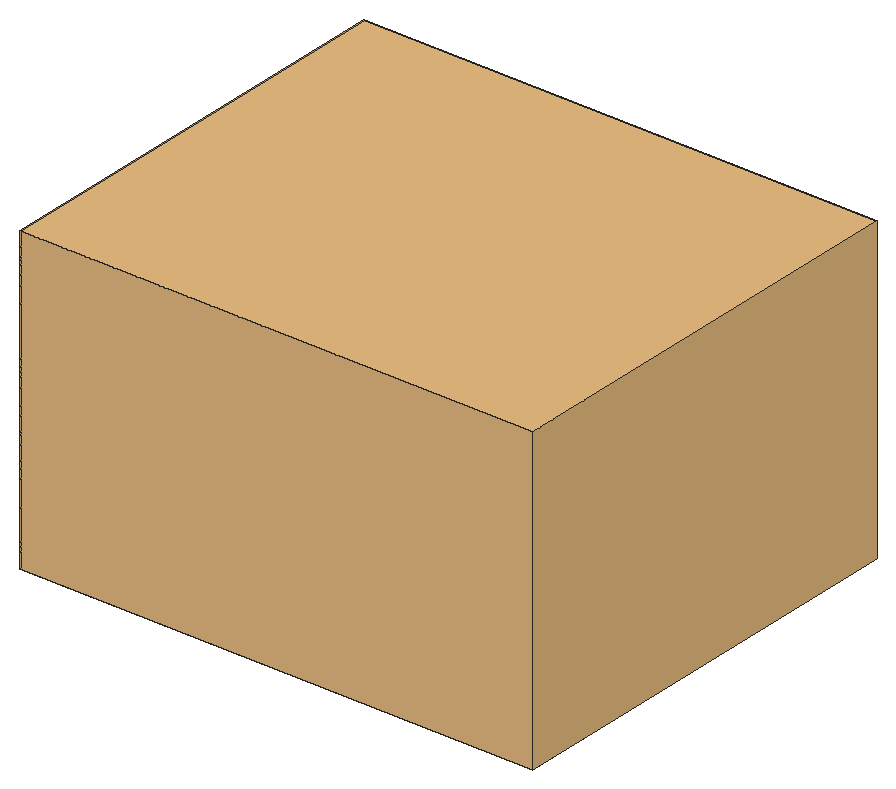
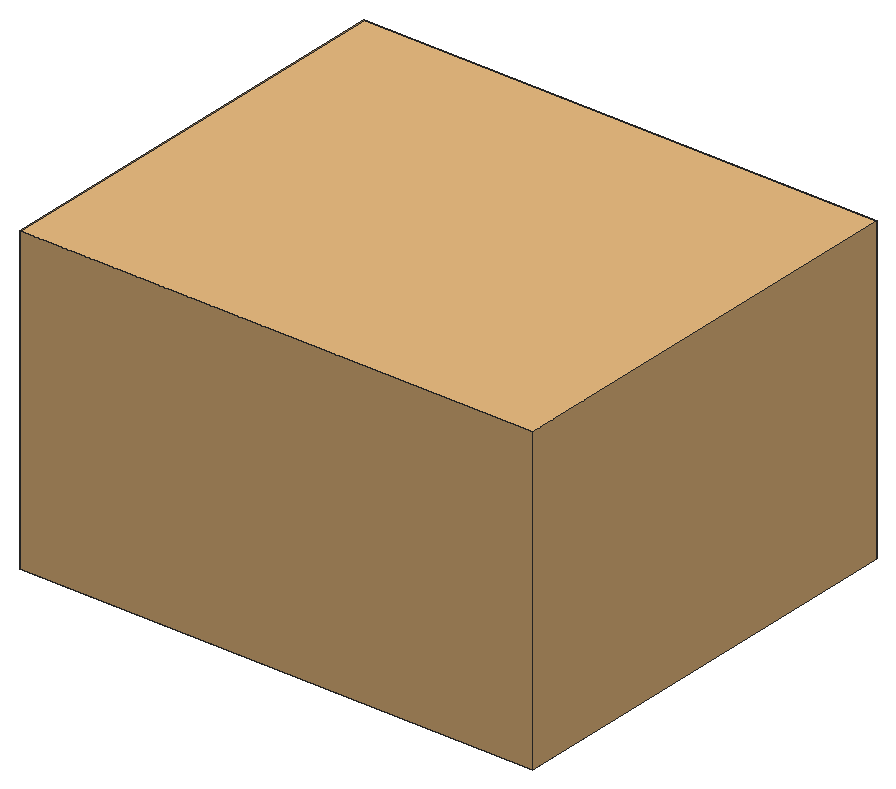
# SketchUp Ruby script. Lengths in inches.
U = 1.inch
M = Sketchup.active_model
def pt(a) = Geom::Point3d.new(a.map { |v| v * U })
def face(e, loops, mat)
  f = e.add_face(loops[0].map { |a| pt(a) })
  loops[1..].each { |l| e.add_face(l.map { |a| pt(a) }).erase! }
  f.material = f.back_material = mat if mat
  f
end
# faces: each face lists its corners as indices into pts; further lists are holes
def faces(e, pts, list, mat = nil) = list.each { |f| face(e, (f[0].is_a?(Array) ? f : [f]).map { |l| l.map { |i| pts[i] } }, mat) }
# xy, xz, yz: faces in a plane at the given z, y or x. An outline is a flat list of corners, or four numbers for a rectangle; further outlines are holes
def ring(l) = l.size == 4 ? [[l[0], l[1]], [l[2], l[1]], [l[2], l[3]], [l[0], l[3]]] : l.each_slice(2).to_a
def flat(e, list, mat, &to3) = list.each { |f| face(e, (f[0].is_a?(Array) ? f : [f]).map { |l| ring(l).map { |u, v| to3.(u, v) } }, mat) }
def xy(e, z, list, mat = nil) = flat(e, list, mat) { |x, y| [x, y, z] }
def xz(e, y, list, mat = nil) = flat(e, list, mat) { |x, z| [x, y, z] }
def yz(e, x, list, mat = nil) = flat(e, list, mat) { |y, z| [x, y, z] }
def lines(e, pts, list) = list.each { |a, b| e.add_line(pt(pts[a]), pt(pts[b])) }
# prism: a flat outline (further loops are holes) pulled along v
def prism(e, loops, v, mat = nil)
  f = face(e, loops, mat); d = Geom::Vector3d.new(v.map { |x| x * U })
  f.pushpull(f.normal.samedirection?(d) ? d.length : -d.length)
end
def box(e, o, s, mat = nil) = prism(e, [[o, [o[0] + s[0], o[1], o[2]], [o[0] + s[0], o[1] + s[1], o[2]], [o[0], o[1] + s[1], o[2]]]], [0, 0, s[2]], mat)
def at(x, y, z, deg = 0) = Geom::Transformation.translation(pt([x, y, z])) * Geom::Transformation.rotation(ORIGIN, Z_AXIS, deg.degrees)
def axes(o, x, y, z) = Geom::Transformation.new([*x, 0, *y, 0, *z, 0, *pt(o).to_a, 1])
def part(name) = M.definitions.add(name)
# library, detail: a bought-in or finely detailed component or shape, given as its bounding box
def library(name, o, s) = part(name).tap { |d| box(d.entities, o, s) }
def detail(e, o, s) = box(e.add_group.entities, o, s)
def put(e, d, t, mat = nil) = e.add_instance(d, t).tap { |i| i.material = mat if mat }
def group(e, t, mat = nil) = e.add_group.tap { |g| g.transformation = t; g.material = mat if mat }.entities
root = M.entities
M.materials.add("1432 AP 8245 TAR ROAD").color = [57, 57, 60]
c1 = library("Group\#17",[-9,-12.5,-6],[243.5,204.5,144])
xz(root,255.5,[[189.84,108,189.92,111],[189.92,108,190,111],[190,108,190.08,111],[190.08,108,190.16,111],[259.34,108,259.42,111],
  [259.42,108,259.5,111],[259.5,108,259.58,111],[259.58,108,259.66,111]])
xz(root,314,[[259.34,108,259.42,111],[259.42,108,259.5,111],[259.5,108,259.58,111],[259.58,108,259.66,111]])
xz(root,320,[[259.34,108,259.42,111],[259.42,108,259.5,111],[259.5,108,259.58,111],[259.58,108,259.66,111]])
yz(root,193,[[252.34,108,252.42,111],[252.42,108,252.5,111],[252.5,108,252.58,111],[252.58,108,252.66,111]])
yz(root,213,[[275,107.5,335,108.5]])
yz(root,215,[[273,108,333,108.5]])
yz(root,256.5,[[252.34,108,252.42,111],[252.42,108,252.5,111],[252.5,108,252.58,111],[252.58,108,252.66,111],[316.84,108,316.92,111],
  [316.92,108,317,111],[317,108,317.08,111],[317.08,108,317.16,111]])
p = [[191.76,250.07,108],[191.7,250.03,108],[191.7,250.03,111],[191.76,250.07,111],[191.83,250.12,108],[191.83,250.12,111],
  [191.89,250.17,108],[191.89,250.17,111],[257.67,250.12,108],[257.61,250.17,108],[257.61,250.17,111],[257.67,250.12,111],
  [257.74,250.07,108],[257.74,250.07,111],[191.95,250.22,108],[191.95,250.22,111],[192.01,250.27,108],[192.01,250.27,111],
  [257.55,250.22,108],[257.49,250.27,108],[257.49,250.27,111],[257.55,250.22,111],[192.07,250.32,108],[192.07,250.32,111],
  [192.12,250.38,108],[192.12,250.38,111],[257.43,250.32,108],[257.43,250.32,111],[257.38,250.38,108],[257.38,250.38,111],
  [192.18,250.43,108],[192.18,250.43,111],[192.23,250.49,108],[192.23,250.49,111],[257.32,250.43,108],[257.32,250.43,111],
  [257.27,250.49,108],[257.27,250.49,111],[192.28,250.55,108],[192.28,250.55,111],[257.22,250.55,108],[257.22,250.55,111],
  [192.33,250.61,108],[192.33,250.61,111],[192.38,250.67,108],[192.38,250.67,111],[257.17,250.61,108],[257.12,250.67,108],
  [257.12,250.67,111],[257.17,250.61,111],[192.43,250.74,108],[192.43,250.74,111],[192.47,250.8,108],[192.47,250.8,111],
  [257.07,250.74,108],[257.03,250.8,108],[257.03,250.8,111],[257.07,250.74,111],[192.52,250.87,108],[192.52,250.87,111],
  [256.98,250.87,108],[256.98,250.87,111],[192.56,250.93,108],[192.56,250.93,111],[192.6,251,108],[192.6,251,111],
  [256.94,250.93,108],[256.94,250.93,111],[256.9,251,108],[256.9,251,111],[192.64,251.07,108],[192.64,251.07,111],
  [256.86,251.07,108],[256.86,251.07,111],[192.67,251.14,108],[192.67,251.14,111],[192.71,251.21,108],[192.71,251.21,111],
  [256.83,251.14,108],[256.83,251.14,111],[256.79,251.21,108],[256.79,251.21,111],[192.74,251.28,108],[192.74,251.28,111],
  [256.76,251.28,108],[256.76,251.28,111],[192.77,251.35,108],[192.77,251.35,111],[256.73,251.35,108],[256.73,251.35,111],
  [192.8,251.42,108],[192.8,251.42,111],[192.83,251.5,108],[192.83,251.5,111],[256.7,251.42,108],[256.7,251.42,111],
  [256.67,251.5,108],[256.67,251.5,111],[192.85,251.57,108],[192.85,251.57,111],[256.65,251.57,108],[256.65,251.57,111],
  [192.875,251.65,108],[192.875,251.65,111],[192.9,251.72,108],[192.9,251.72,111],[256.625,251.65,108],[256.625,251.65,111],
  [256.6,251.72,108],[256.6,251.72,111],[192.92,251.8,108],[192.92,251.8,111],[256.58,251.8,108],[256.58,251.8,111],
  [192.93,251.875,108],[192.93,251.875,111],[256.57,251.875,108],[256.57,251.875,111],[192.95,251.95,108],[192.95,251.95,111],
  [256.55,251.95,108],[256.55,251.95,111],[192.96,252.03,108],[192.96,252.03,111],[192.97,252.11,108],[192.97,252.11,111],
  [256.54,252.03,108],[256.54,252.03,111],[256.53,252.11,108],[256.53,252.11,111],[192.98,252.1875,108],[192.98,252.1875,111],
  [256.52,252.1875,108],[256.52,252.1875,111],[192.99,252.26,108],[192.99,252.26,111],[256.51,252.26,108],[256.51,252.26,111],
  [193,252.34,108],[193,252.34,111],[256.5,252.34,108],[256.5,252.34,111],[192.99,252.74,108],[193,252.66,108],
  [193,252.66,111],[192.99,252.74,111],[192.98,252.8125,108],[192.98,252.8125,111],[256.5,252.66,108],[256.51,252.74,108],
  [256.51,252.74,111],[256.5,252.66,111],[256.52,252.8125,108],[256.52,252.8125,111],[192.97,252.89,108],[192.97,252.89,111],
  [256.53,252.89,108],[256.53,252.89,111],[192.96,252.97,108],[192.96,252.97,111],[256.54,252.97,108],[256.54,252.97,111],
  [192.95,253.05,108],[192.95,253.05,111],[192.93,253.125,108],[192.93,253.125,111],[256.55,253.05,108],[256.55,253.05,111],
  [256.57,253.125,108],[256.57,253.125,111],[192.92,253.2,108],[192.92,253.2,111],[256.58,253.2,108],[256.58,253.2,111],
  [192.9,253.28,108],[192.9,253.28,111],[256.6,253.28,108],[256.6,253.28,111],[192.875,253.35,108],[192.875,253.35,111],
  [256.625,253.35,108],[256.625,253.35,111],[192.83,253.5,108],[192.85,253.43,108],[192.85,253.43,111],[192.83,253.5,111],
  [256.65,253.43,108],[256.65,253.43,111],[256.67,253.5,108],[256.67,253.5,111],[192.8,253.58,108],[192.8,253.58,111],
  [256.7,253.58,108],[256.7,253.58,111],[192.74,253.72,108],[192.77,253.65,108],[192.77,253.65,111],[192.74,253.72,111],
  [256.73,253.65,108],[256.73,253.65,111],[256.76,253.72,108],[256.76,253.72,111],[192.71,253.79,108],[192.71,253.79,111],
  [256.79,253.79,108],[256.79,253.79,111],[192.67,253.86,108],[192.67,253.86,111],[256.83,253.86,108],[256.83,253.86,111],
  [192.64,253.93,108],[192.64,253.93,111],[192.6,254,108],[192.6,254,111],[256.86,253.93,108],[256.86,253.93,111],
  [256.9,254,108],[256.9,254,111],[192.56,254.07,108],[192.56,254.07,111],[256.94,254.07,108],[256.94,254.07,111],
  [192.52,254.13,108],[192.52,254.13,111],[192.47,254.2,108],[192.47,254.2,111],[256.98,254.13,108],[256.98,254.13,111],
  [257.03,254.2,108],[257.03,254.2,111],[192.43,254.26,108],[192.43,254.26,111],[257.07,254.26,108],[257.07,254.26,111],
  [192.33,254.39,108],[192.38,254.33,108],[192.38,254.33,111],[192.33,254.39,111],[257.12,254.33,108],[257.12,254.33,111],
  [257.17,254.39,108],[257.17,254.39,111],[192.23,254.51,108],[192.28,254.45,108],[192.28,254.45,111],[192.23,254.51,111],
  [257.22,254.45,108],[257.22,254.45,111],[257.27,254.51,108],[257.27,254.51,111],[192.18,254.57,108],[192.18,254.57,111],
  [257.32,254.57,108],[257.32,254.57,111],[192.12,254.62,108],[192.12,254.62,111],[192.07,254.68,108],[192.07,254.68,111],
  [257.38,254.62,108],[257.38,254.62,111],[257.43,254.68,108],[257.43,254.68,111],[191.95,254.78,108],[192.01,254.73,108],
  [192.01,254.73,111],[191.95,254.78,111],[257.49,254.73,108],[257.49,254.73,111],[257.55,254.78,108],[257.55,254.78,111],
  [191.83,254.88,108],[191.89,254.83,108],[191.89,254.83,111],[191.83,254.88,111],[257.61,254.83,108],[257.61,254.83,111],
  [257.67,254.88,108],[257.67,254.88,111],[191.7,254.97,108],[191.76,254.93,108],[191.76,254.93,111],[191.7,254.97,111],
  [257.74,254.93,108],[257.74,254.93,111],[257.8,254.97,108],[257.8,254.97,111],[191.63,255.02,108],[191.63,255.02,111],
  [191.57,255.06,108],[191.57,255.06,111],[257.87,255.02,108],[257.87,255.02,111],[257.93,255.06,108],[257.93,255.06,111],
  [191.43,255.14,108],[191.5,255.1,108],[191.5,255.1,111],[191.43,255.14,111],[191.36,255.17,108],[191.36,255.17,111],
  [258,255.1,108],[258,255.1,111],[258.07,255.14,108],[258.07,255.14,111],[258.14,255.17,108],[258.14,255.17,111],
  [191.15,255.27,108],[191.22,255.24,108],[191.22,255.24,111],[191.15,255.27,111],[191.29,255.21,108],[191.29,255.21,111],
  [258.21,255.21,108],[258.21,255.21,111],[258.28,255.24,108],[258.28,255.24,111],[258.35,255.27,108],[258.35,255.27,111],
  [190.93,255.35,108],[191,255.33,108],[191,255.33,111],[190.93,255.35,111],[191.08,255.3,108],[191.08,255.3,111],
  [258.42,255.3,108],[258.42,255.3,111],[258.5,255.33,108],[258.5,255.33,111],[258.57,255.35,108],[258.57,255.35,111],
  [189.15,255.375,108],[189.22,255.4,108],[189.22,255.4,111],[189.15,255.375,111],[189.3,255.42,108],[189.3,255.42,111],
  [189.375,255.43,108],[189.375,255.43,111],[189.45,255.45,108],[189.45,255.45,111],[189.53,255.46,108],[189.53,255.46,111],
  [190.55,255.45,108],[190.625,255.43,108],[190.625,255.43,111],[190.55,255.45,111],[190.47,255.46,108],[190.47,255.46,111],
  [190.7,255.42,108],[190.7,255.42,111],[190.78,255.4,108],[190.78,255.4,111],[190.85,255.375,108],[190.85,255.375,111],
  [258.65,255.375,108],[258.65,255.375,111],[258.72,255.4,108],[258.72,255.4,111],[258.8,255.42,108],[258.8,255.42,111],
  [258.875,255.43,108],[258.875,255.43,111],[258.95,255.45,108],[258.95,255.45,111],[259.03,255.46,108],[259.03,255.46,111],
  [189.61,255.47,108],[189.61,255.47,111],[189.6875,255.48,108],[189.6875,255.48,111],[189.76,255.49,108],[189.76,255.49,111],
  [189.84,255.5,108],[189.84,255.5,111],[190.24,255.49,108],[190.3125,255.48,108],[190.3125,255.48,111],[190.24,255.49,111],
  [190.16,255.5,108],[190.16,255.5,111],[190.39,255.47,108],[190.39,255.47,111],[259.11,255.47,108],[259.11,255.47,111],
  [259.1875,255.48,108],[259.1875,255.48,111],[259.26,255.49,108],[259.26,255.49,111],[259.34,255.5,108],[259.34,255.5,111],
  [259.74,255.49,108],[259.8125,255.48,108],[259.8125,255.48,111],[259.74,255.49,111],[259.66,255.5,108],[259.66,255.5,111],
  [259.89,255.47,108],[259.89,255.47,111],[259.97,255.46,108],[259.97,255.46,111],[259.11,314.03,108],[259.03,314.04,108],
  [259.03,314.04,111],[259.11,314.03,111],[258.95,314.05,108],[258.95,314.05,111],[259.1875,314.02,108],[259.1875,314.02,111],
  [259.26,314.01,108],[259.26,314.01,111],[259.34,314,108],[259.34,314,111],[259.74,314.01,108],[259.66,314,108],
  [259.66,314,111],[259.74,314.01,111],[259.8125,314.02,108],[259.8125,314.02,111],[259.89,314.03,108],[259.89,314.03,111],
  [258.57,314.15,108],[258.5,314.17,108],[258.5,314.17,111],[258.57,314.15,111],[258.72,314.1,108],[258.65,314.125,108],
  [258.65,314.125,111],[258.72,314.1,111],[258.8,314.08,108],[258.8,314.08,111],[258.875,314.07,108],[258.875,314.07,111],
  [258.35,314.23,108],[258.28,314.26,108],[258.28,314.26,111],[258.35,314.23,111],[258.42,314.2,108],[258.42,314.2,111],
  [258.21,314.29,108],[258.14,314.33,108],[258.14,314.33,111],[258.21,314.29,111],[258.07,314.36,108],[258.07,314.36,111],
  [258,314.4,108],[257.93,314.44,108],[257.93,314.44,111],[258,314.4,111],[257.87,314.48,108],[257.87,314.48,111],
  [257.8,314.53,108],[257.74,314.57,108],[257.74,314.57,111],[257.8,314.53,111],[257.67,314.62,108],[257.61,314.67,108],
  [257.61,314.67,111],[257.67,314.62,111],[257.55,314.72,108],[257.49,314.77,108],[257.49,314.77,111],[257.55,314.72,111],
  [257.43,314.82,108],[257.43,314.82,111],[257.38,314.88,108],[257.38,314.88,111],[257.32,314.93,108],[257.32,314.93,111],
  [257.27,314.99,108],[257.27,314.99,111],[257.22,315.05,108],[257.22,315.05,111],[257.17,315.11,108],[257.12,315.17,108],
  [257.12,315.17,111],[257.17,315.11,111],[257.07,315.24,108],[257.03,315.3,108],[257.03,315.3,111],[257.07,315.24,111],
  [256.98,315.37,108],[256.98,315.37,111],[256.94,315.43,108],[256.94,315.43,111],[256.9,315.5,108],[256.9,315.5,111],
  [256.86,315.57,108],[256.86,315.57,111],[256.83,315.64,108],[256.83,315.64,111],[256.79,315.71,108],[256.79,315.71,111],
  [256.76,315.78,108],[256.76,315.78,111],[256.73,315.85,108],[256.73,315.85,111],[256.7,315.92,108],[256.7,315.92,111],
  [256.67,316,108],[256.67,316,111],[256.65,316.07,108],[256.65,316.07,111],[256.625,316.15,108],[256.625,316.15,111],
  [256.6,316.22,108],[256.6,316.22,111],[256.58,316.3,108],[256.58,316.3,111],[256.57,316.375,108],[256.57,316.375,111],
  [256.55,316.45,108],[256.55,316.45,111],[256.54,316.53,108],[256.54,316.53,111],[256.53,316.61,108],[256.53,316.61,111],
  [256.52,316.6875,108],[256.52,316.6875,111],[256.51,316.76,108],[256.51,316.76,111],[256.5,316.84,108],[256.5,316.84,111],
  [256.5,317.16,108],[256.51,317.24,108],[256.51,317.24,111],[256.5,317.16,111],[256.52,317.3125,108],[256.52,317.3125,111],
  [256.53,317.39,108],[256.53,317.39,111],[256.54,317.47,108],[256.54,317.47,111],[256.55,317.55,108],[256.55,317.55,111],
  [256.57,317.625,108],[256.57,317.625,111],[256.58,317.7,108],[256.58,317.7,111],[256.6,317.78,108],[256.6,317.78,111],
  [256.625,317.85,108],[256.625,317.85,111],[256.65,317.93,108],[256.65,317.93,111],[256.67,318,108],[256.67,318,111],
  [256.7,318.08,108],[256.7,318.08,111],[256.73,318.15,108],[256.73,318.15,111],[256.76,318.22,108],[256.76,318.22,111],
  [256.79,318.29,108],[256.79,318.29,111],[256.83,318.36,108],[256.83,318.36,111],[256.86,318.43,108],[256.86,318.43,111],
  [256.9,318.5,108],[256.9,318.5,111],[256.94,318.57,108],[256.94,318.57,111],[256.98,318.63,108],[256.98,318.63,111],
  [257.03,318.7,108],[257.03,318.7,111],[257.07,318.76,108],[257.07,318.76,111],[257.12,318.83,108],[257.12,318.83,111],
  [257.17,318.89,108],[257.17,318.89,111],[257.22,318.95,108],[257.22,318.95,111],[257.27,319.01,108],[257.27,319.01,111],
  [257.32,319.07,108],[257.32,319.07,111],[257.38,319.12,108],[257.38,319.12,111],[257.43,319.18,108],[257.43,319.18,111],
  [257.49,319.23,108],[257.49,319.23,111],[257.55,319.28,108],[257.55,319.28,111],[257.61,319.33,108],[257.61,319.33,111],
  [257.67,319.38,108],[257.67,319.38,111],[257.74,319.43,108],[257.74,319.43,111],[257.8,319.47,108],[257.8,319.47,111],
  [257.87,319.52,108],[257.87,319.52,111],[257.93,319.56,108],[257.93,319.56,111],[258,319.6,108],[258,319.6,111],
  [258.07,319.64,108],[258.07,319.64,111],[258.14,319.67,108],[258.14,319.67,111],[258.21,319.71,108],[258.21,319.71,111],
  [258.28,319.74,108],[258.28,319.74,111],[258.35,319.77,108],[258.35,319.77,111],[258.42,319.8,108],[258.42,319.8,111],
  [258.5,319.83,108],[258.5,319.83,111],[258.57,319.85,108],[258.57,319.85,111],[258.65,319.875,108],[258.65,319.875,111],
  [258.72,319.9,108],[258.72,319.9,111],[258.8,319.92,108],[258.8,319.92,111],[258.875,319.93,108],[258.875,319.93,111],
  [258.95,319.95,108],[258.95,319.95,111],[259.03,319.96,108],[259.03,319.96,111],[259.11,319.97,108],[259.11,319.97,111],
  [259.1875,319.98,108],[259.1875,319.98,111],[259.26,319.99,108],[259.26,319.99,111],[259.34,320,108],[259.34,320,111],
  [259.74,319.99,108],[259.8125,319.98,108],[259.8125,319.98,111],[259.74,319.99,111],[259.66,320,108],[259.66,320,111],
  [259.89,319.97,108],[259.89,319.97,111]]
faces(root,p,[[0,1,2,3],[4,0,3,5],[6,4,5,7],[8,9,10,11],[12,8,11,13],[14,6,7,15],[16,14,15,17],[18,19,20,21],
  [9,18,21,10],[22,16,17,23],[24,22,23,25],[19,26,27,20],[26,28,29,27],[30,24,25,31],[32,30,31,33],[28,34,35,29],
  [34,36,37,35],[38,32,33,39],[36,40,41,37],[42,38,39,43],[44,42,43,45],[46,47,48,49],[40,46,49,41],[50,44,45,51],
  [52,50,51,53],[54,55,56,57],[47,54,57,48],[58,52,53,59],[55,60,61,56],[62,58,59,63],[64,62,63,65],[60,66,67,61],
  [66,68,69,67],[70,64,65,71],[68,72,73,69],[74,70,71,75],[76,74,75,77],[72,78,79,73],[78,80,81,79],[82,76,77,83],
  [80,84,85,81],[86,82,83,87],[84,88,89,85],[90,86,87,91],[92,90,91,93],[88,94,95,89],[94,96,97,95],[98,92,93,99],
  [96,100,101,97],[102,98,99,103],[104,102,103,105],[100,106,107,101],[106,108,109,107],[110,104,105,111],[108,112,113,109],[114,110,111,115],
  [112,116,117,113],[118,114,115,119],[116,120,121,117],[122,118,119,123],[124,122,123,125],[120,126,127,121],[126,128,129,127],[130,124,125,131],
  [128,132,133,129],[134,130,131,135],[132,136,137,133],[138,134,135,139],[136,140,141,137],[142,143,144,145],[146,142,145,147],[148,149,150,151],
  [149,152,153,150],[154,146,147,155],[152,156,157,153],[158,154,155,159],[156,160,161,157],[162,158,159,163],[164,162,163,165],[160,166,167,161],
  [166,168,169,167],[170,164,165,171],[168,172,173,169],[174,170,171,175],[172,176,177,173],[178,174,175,179],[176,180,181,177],[182,183,184,185],
  [183,178,179,184],[180,186,187,181],[186,188,189,187],[190,182,185,191],[188,192,193,189],[194,195,196,197],[195,190,191,196],[192,198,199,193],
  [198,200,201,199],[202,194,197,203],[200,204,205,201],[206,202,203,207],[204,208,209,205],[210,206,207,211],[212,210,211,213],[208,214,215,209],
  [214,216,217,215],[218,212,213,219],[216,220,221,217],[222,218,219,223],[224,222,223,225],[220,226,227,221],[226,228,229,227],[230,224,225,231],
  [228,232,233,229],[234,235,236,237],[235,230,231,236],[232,238,239,233],[238,240,241,239],[242,243,244,245],[243,234,237,244],[240,246,247,241],
  [246,248,249,247],[250,242,245,251],[248,252,253,249],[254,250,251,255],[256,254,255,257],[252,258,259,253],[258,260,261,259],[262,263,264,265],
  [263,256,257,264],[260,266,267,261],[266,268,269,267],[270,271,272,273],[271,262,265,272],[268,274,275,269],[274,276,277,275],[278,279,280,281],
  [279,270,273,280],[276,282,283,277],[282,284,285,283],[286,278,281,287],[288,286,287,289],[284,290,291,285],[290,292,293,291],[294,295,296,297],
  [298,294,297,299],[295,288,289,296],[292,300,301,293],[300,302,303,301],[302,304,305,303],[306,307,308,309],[307,310,311,308],[310,298,299,311],
  [304,312,313,305],[312,314,315,313],[314,316,317,315],[318,319,320,321],[319,322,323,320],[322,306,309,323],[316,324,325,317],[324,326,327,325],
  [326,328,329,327],[330,331,332,333],[331,334,335,332],[334,336,337,335],[336,338,339,337],[338,340,341,339],[342,343,344,345],[346,342,345,347],
  [343,348,349,344],[348,350,351,349],[350,352,353,351],[352,318,321,353],[328,354,355,329],[354,356,357,355],[356,358,359,357],[358,360,361,359],
  [360,362,363,361],[362,364,365,363],[340,366,367,341],[366,368,369,367],[368,370,371,369],[370,372,373,371],[374,375,376,377],[378,374,377,379],
  [375,380,381,376],[380,346,347,381],[364,382,383,365],[382,384,385,383],[384,386,387,385],[386,388,389,387],[390,391,392,393],[394,390,393,395],
  [391,396,397,392],[396,398,399,397],[400,401,402,403],[401,404,405,402],[406,400,403,407],[408,406,407,409],[410,408,409,411],[412,413,414,415],
  [416,412,415,417],[418,416,417,419],[420,421,422,423],[424,425,426,427],[425,420,423,426],[428,424,427,429],[430,428,429,431],[404,430,431,405],
  [432,433,434,435],[421,436,437,422],[436,432,435,437],[438,439,440,441],[439,442,443,440],[433,438,441,434],[444,445,446,447],[445,448,449,446],
  [442,444,447,443],[450,451,452,453],[448,450,453,449],[454,455,456,457],[451,454,457,452],[458,459,460,461],[455,458,461,456],[459,462,463,460],
  [462,464,465,463],[464,466,467,465],[466,468,469,467],[468,470,471,469],[472,473,474,475],[470,472,475,471],[476,477,478,479],[473,476,479,474],
  [477,480,481,478],[480,482,483,481],[482,484,485,483],[484,486,487,485],[486,488,489,487],[488,490,491,489],[490,492,493,491],[492,494,495,493],
  [494,496,497,495],[496,498,499,497],[498,500,501,499],[500,502,503,501],[502,504,505,503],[504,506,507,505],[506,508,509,507],[508,510,511,509],
  [510,512,513,511],[512,514,515,513],[514,516,517,515],[516,518,519,517],[518,520,521,519],[522,523,524,525],[523,526,527,524],[526,528,529,527],
  [528,530,531,529],[530,532,533,531],[532,534,535,533],[534,536,537,535],[536,538,539,537],[538,540,541,539],[540,542,543,541],[542,544,545,543],
  [544,546,547,545],[546,548,549,547],[548,550,551,549],[550,552,553,551],[552,554,555,553],[554,556,557,555],[556,558,559,557],[558,560,561,559],
  [560,562,563,561],[562,564,565,563],[564,566,567,565],[566,568,569,567],[568,570,571,569],[570,572,573,571],[572,574,575,573],[574,576,577,575],
  [576,578,579,577],[578,580,581,579],[580,582,583,581],[582,584,585,583],[584,586,587,585],[586,588,589,587],[588,590,591,589],[590,592,593,591],
  [592,594,595,593],[594,596,597,595],[596,598,599,597],[598,600,601,599],[600,602,603,601],[602,604,605,603],[604,606,607,605],[606,608,609,607],
  [608,610,611,609],[610,612,613,611],[612,614,615,613],[614,616,617,615],[616,618,619,617],[618,620,621,619],[620,622,623,621],[622,624,625,623],
  [624,626,627,625],[626,628,629,627],[628,630,631,629],[630,632,633,631],[632,634,635,633],[636,637,638,639],[640,636,639,641],[637,642,643,638]])
put(root,c1,at(120,164,114),"1432 AP 8245 TAR ROAD")
